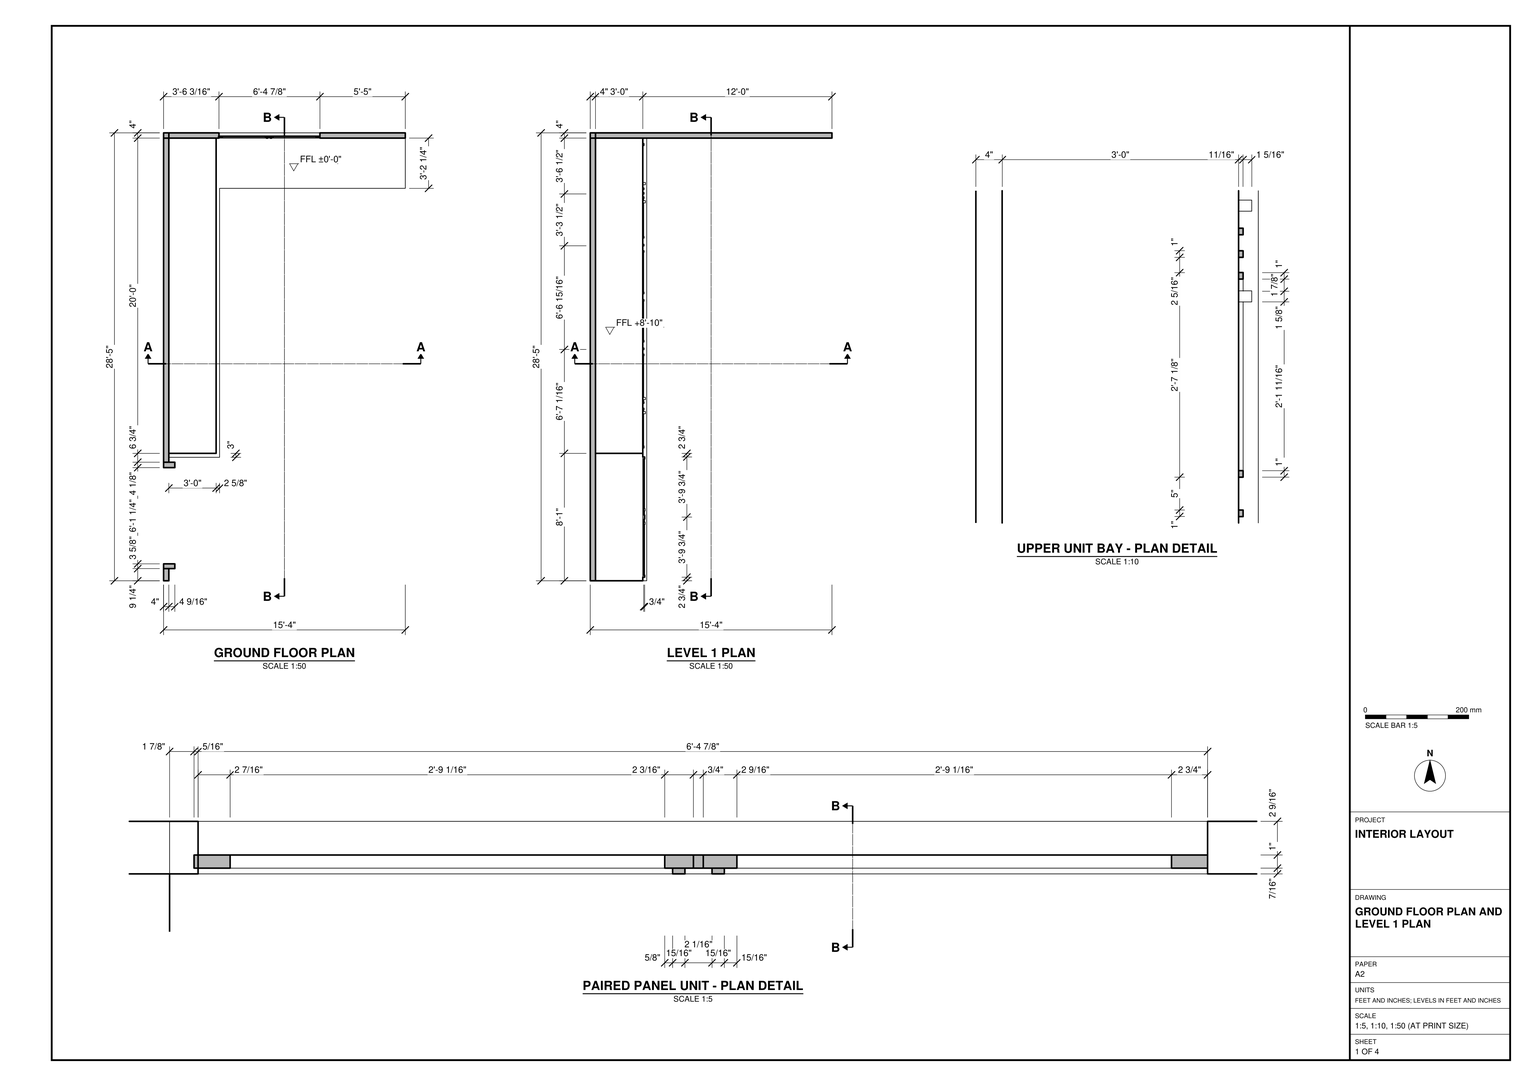
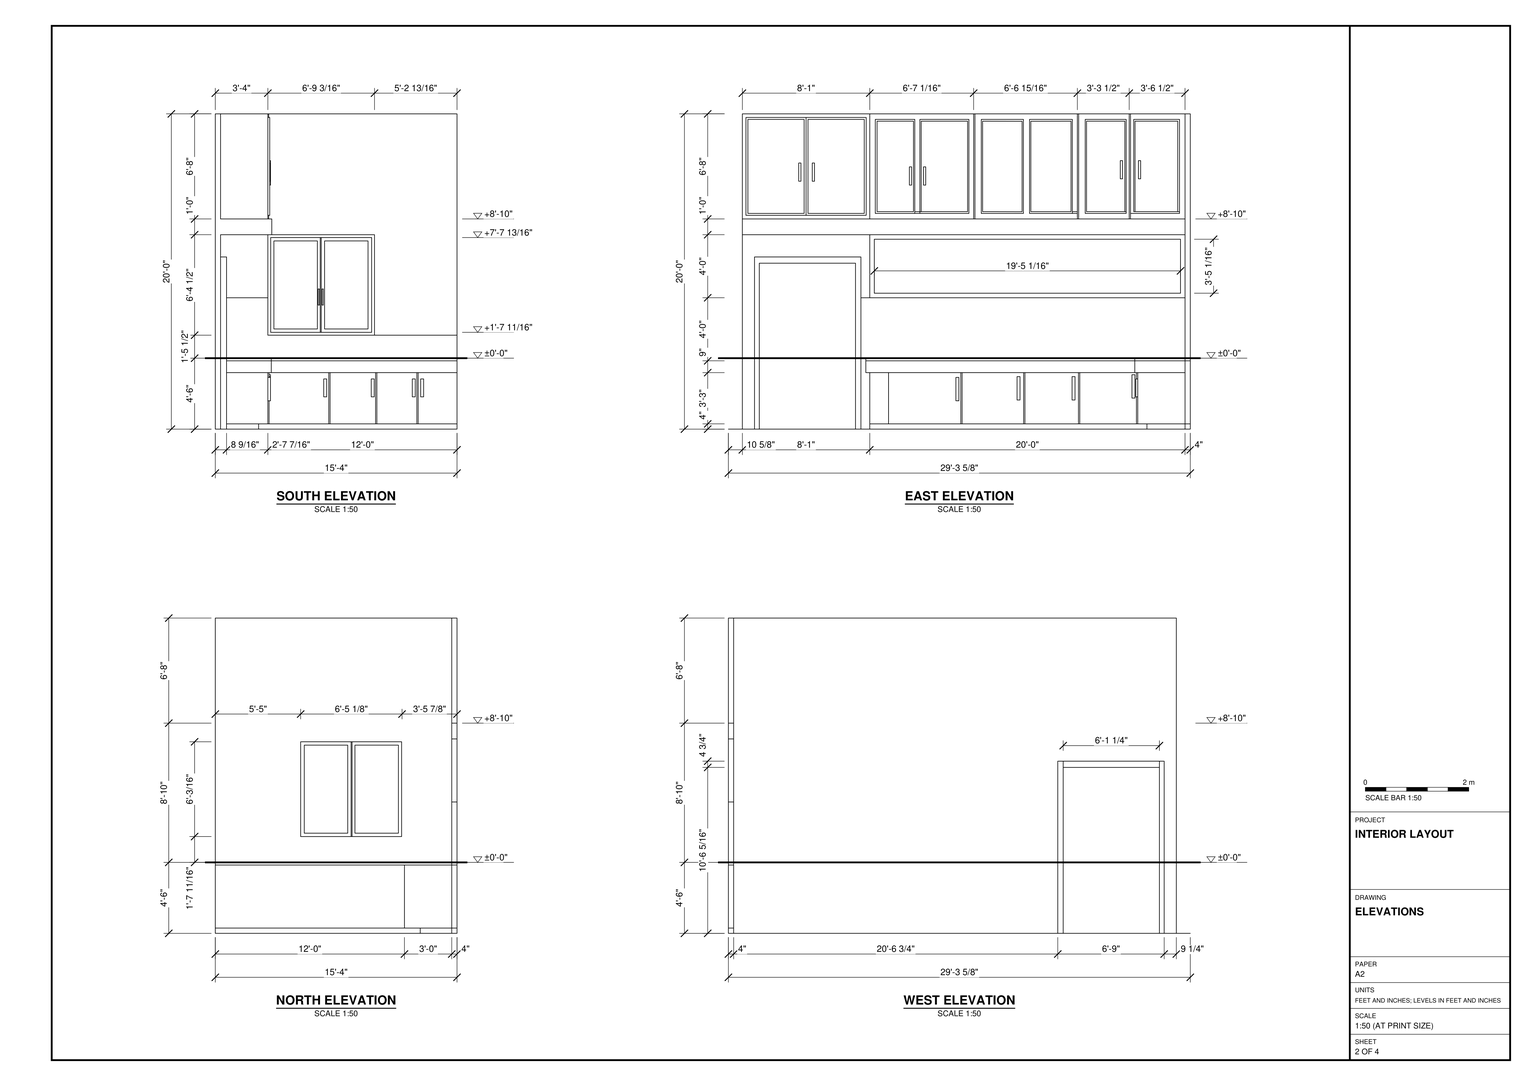
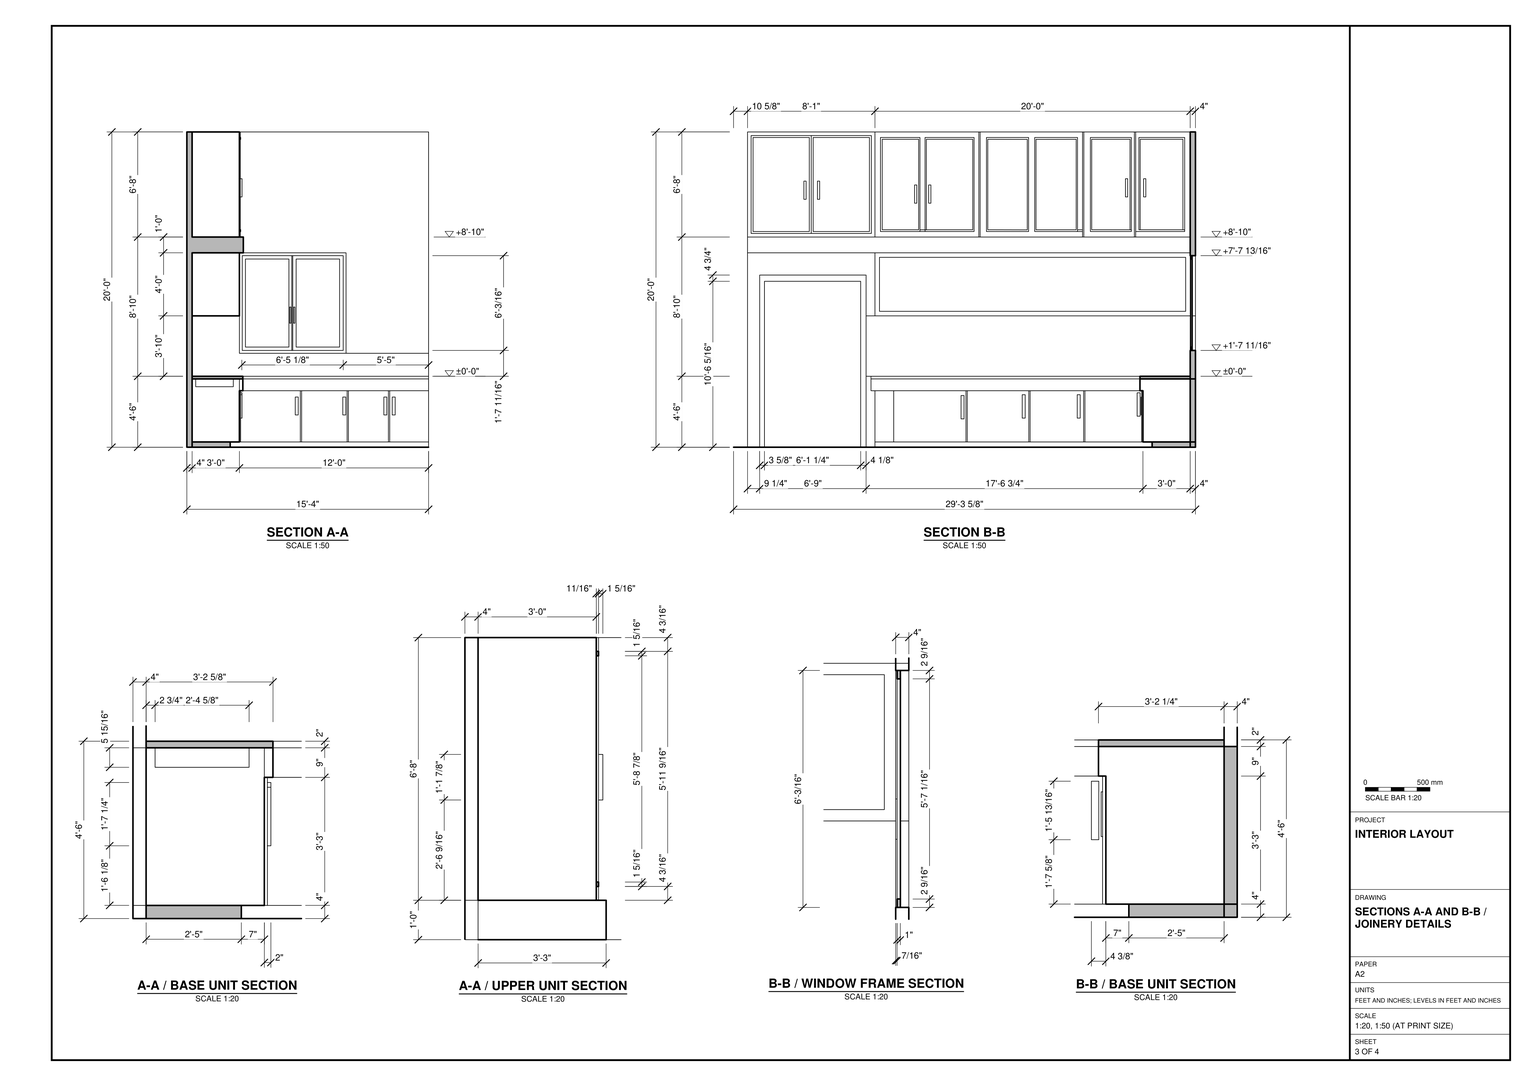
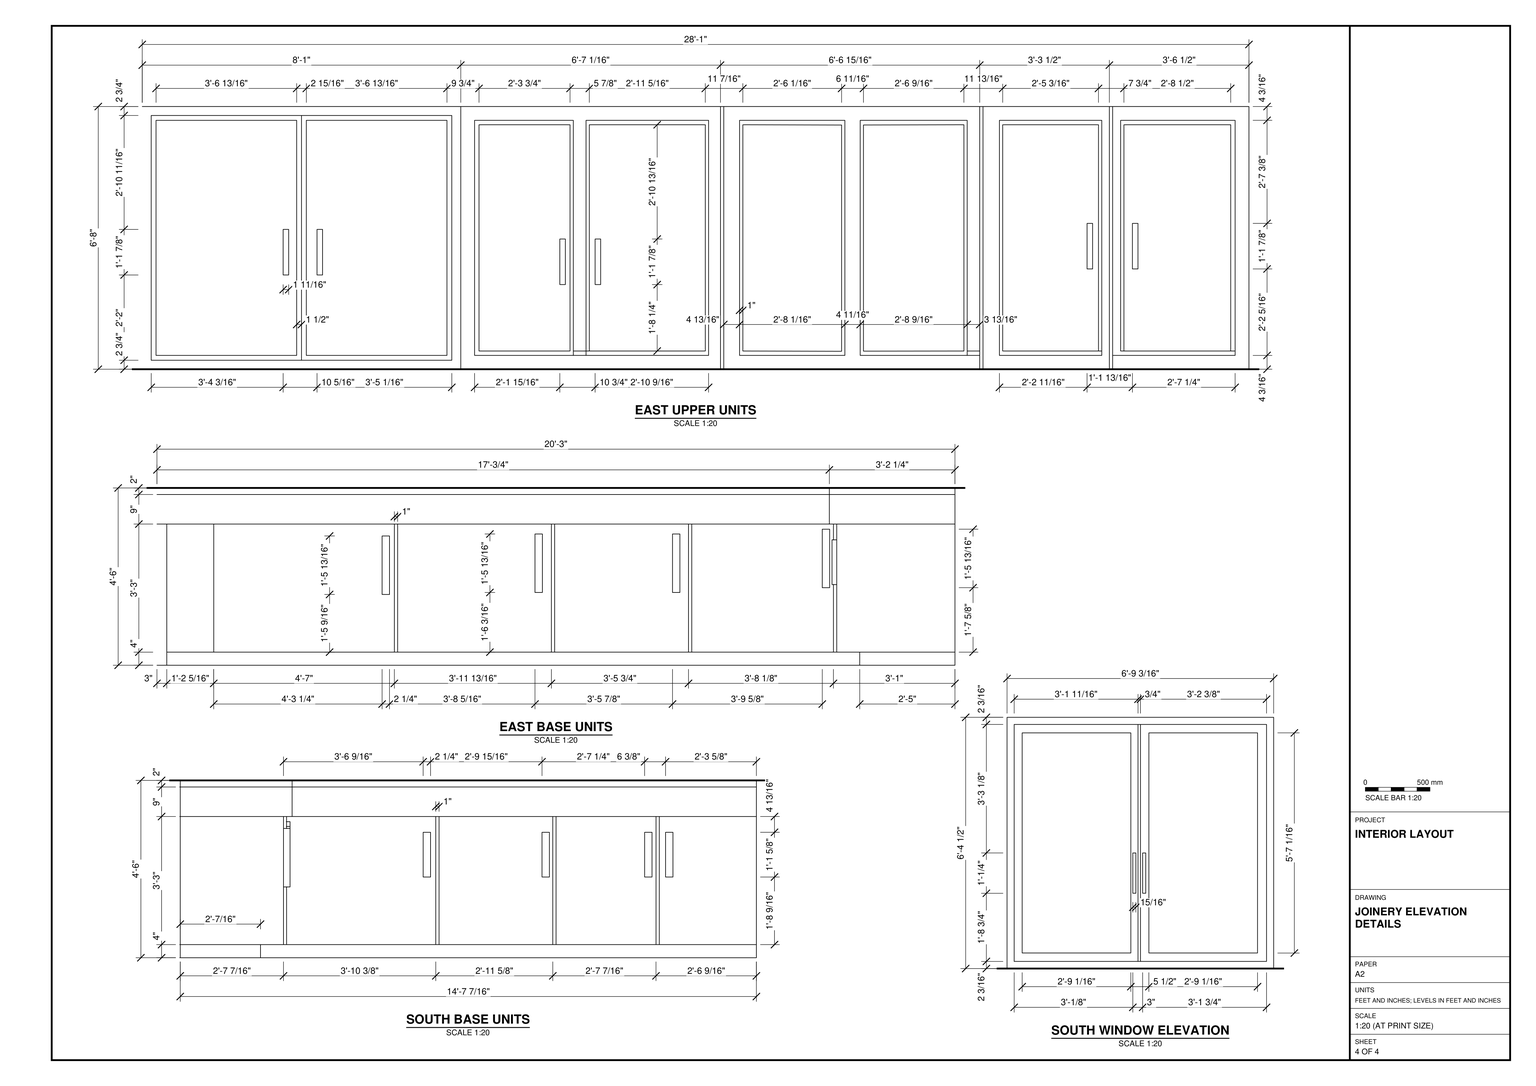
Build the interior fit-out in SketchUp from task_files/diagram_01.pdf. Work in feet and inches. Set the overall width to 15'-4", depth to 29'-3 5/8", and height to 20'-0". Use ±0'-0" as the ground-floor datum and +8'-10" as the Level 1 datum. The ground-floor datum aligns with the worktop, not the bottom of the model: the base units extend 4'-6" below it.

Form the corner with the two perpendicular 4" walls shown in plan. Fit the paired framed window in the short wall above the worktop. On the long wall, leave the tall framed opening near the free end and place the long horizontal framed panel above the base cabinets. Turn the worktop and base units around the inside corner, following the sections for the top overhangs and recessed plinths. Above the long wall run, model the projecting support slab and the upper cabinets. Use the east elevation to lay out the cabinet bays, framed fronts and pulls rather than dividing the run into equal bays.

Keep shell elements such as walls and slabs separate from one another, make each joinery or furniture piece a separate group or component, and use components for repeated parts. Any decor or loose items may be suitable library components. Save one SketchUp model as output_files/l_shaped_interior_fit_out_with_base_and_upper_cabinets.skp.

# SketchUp Ruby script. Lengths in inches.
U = 1.inch
M = Sketchup.active_model
def pt(a) = Geom::Point3d.new(a.map { |v| v * U })
def face(e, loops, mat)
  f = e.add_face(loops[0].map { |a| pt(a) })
  loops[1..].each { |l| e.add_face(l.map { |a| pt(a) }).erase! }
  f.material = f.back_material = mat if mat
  f
end
# faces: each face lists its corners as indices into pts; further lists are holes
def faces(e, pts, list, mat = nil) = list.each { |f| face(e, (f[0].is_a?(Array) ? f : [f]).map { |l| l.map { |i| pts[i] } }, mat) }
# xy, xz, yz: faces in a plane at the given z, y or x. An outline is a flat list of corners, or four numbers for a rectangle; further outlines are holes
def ring(l) = l.size == 4 ? [[l[0], l[1]], [l[2], l[1]], [l[2], l[3]], [l[0], l[3]]] : l.each_slice(2).to_a
def flat(e, list, mat, &to3) = list.each { |f| face(e, (f[0].is_a?(Array) ? f : [f]).map { |l| ring(l).map { |u, v| to3.(u, v) } }, mat) }
def xy(e, z, list, mat = nil) = flat(e, list, mat) { |x, y| [x, y, z] }
def xz(e, y, list, mat = nil) = flat(e, list, mat) { |x, z| [x, y, z] }
def yz(e, x, list, mat = nil) = flat(e, list, mat) { |y, z| [x, y, z] }
def lines(e, pts, list) = list.each { |a, b| e.add_line(pt(pts[a]), pt(pts[b])) }
# prism: a flat outline (further loops are holes) pulled along v
def prism(e, loops, v, mat = nil)
  f = face(e, loops, mat); d = Geom::Vector3d.new(v.map { |x| x * U })
  f.pushpull(f.normal.samedirection?(d) ? d.length : -d.length)
end
def box(e, o, s, mat = nil) = prism(e, [[o, [o[0] + s[0], o[1], o[2]], [o[0] + s[0], o[1] + s[1], o[2]], [o[0], o[1] + s[1], o[2]]]], [0, 0, s[2]], mat)
def at(x, y, z, deg = 0) = Geom::Transformation.translation(pt([x, y, z])) * Geom::Transformation.rotation(ORIGIN, Z_AXIS, deg.degrees)
def axes(o, x, y, z) = Geom::Transformation.new([*x, 0, *y, 0, *z, 0, *pt(o).to_a, 1])
def part(name) = M.definitions.add(name)
# library, detail: a bought-in or finely detailed component or shape, given as its bounding box
def library(name, o, s) = part(name).tap { |d| box(d.entities, o, s) }
def detail(e, o, s) = box(e.add_group.entities, o, s)
def put(e, d, t, mat = nil) = e.add_instance(d, t).tap { |i| i.material = mat if mat }
def group(e, t, mat = nil) = e.add_group.tap { |g| g.transformation = t; g.material = mat if mat }.entities
root = M.entities
M.materials.add("[0123_DarkMagenta]").color = [119, 35, 134]
M.materials.add("[Color C08]").color = [102, 51, 0]
M.materials.add("[Color K08]").color = [81, 11, 69]
M.materials.add("[Color M00]").color = [255, 255, 255]
M.materials.add("[Field Square Tile]").color = [217, 201, 169]
M.materials.add("[Granite Dark Gray]").color = [69, 68, 68]
M.materials.add("[Steel Brushed Stainless]").color = [183, 187, 190]
M.materials.add("[Stone Brushed Khaki]").color = [226, 197, 133]
M.materials.add("[Translucent Glass Gray]").color = [128, 128, 128]
M.materials["[Translucent Glass Gray]"].alpha = 0.5
xy(root,0,[[0,19.89,8.5625,23.52],[0,96.77,8.5625,100.89]])
xy(root,0,[[0,10.625,4,19.89],[0,100.89,4,347.625],[4,107.625,4,347.625,28,347.625,28,323.625,33,323.625,33,107.625],[33,318.625,33,323.625,28,323.625,28,347.625,184,347.625,184,318.625],[0,347.625,4,351.625],
  [4,347.625,28,351.625],[28,347.625,184,351.625]],"[Color M00]")
xy(root,0,[[4,0,4,19.89,8.5625,19.89,8.5625,23.52,0,23.52,0,96.77,8.5625,96.77,8.5625,100.89,4,100.89,4,107.625,33,107.625,33,318.625,184,318.625,184,0]],"[Stone Brushed Khaki]")
xy(root,4,[[33,107.625,40,318.625],[40,176.92,40.9375,177.92],[40,311.625,184,318.625]],"[Color K08]")
xy(root,4,[[4,107.625,4,347.625,28,347.625,28,323.625,33,323.625,33,107.625],[40,224.74,40.9375,225.74],[40,266.49,40.9375,267.49],[86.375,310.625,87.375,311.625],[122,310.625,123,311.625],
  [153.4375,310.625,154.4375,311.625],[33,318.625,33,323.625,28,323.625,28,347.625,40,347.625,40,318.625],[40,318.625,184,347.625],[0,347.625,4,351.625],[4,347.625,28,351.625],
  [28,347.625,40,351.625],[40,347.625,184,351.625]],"[Color M00]")
xy(root,21.56,[[40,173.19,42,175.44]],"[Steel Brushed Stainless]")
xy(root,22.17,[[40,219.74,42,221.99],[40,261.62,42,263.87]],"[Steel Brushed Stainless]")
xy(root,23.62,[[40,307.22,42,309.47]],"[Steel Brushed Stainless]")
xy(root,24.58,[[82.53,310.1875,84.78,311.625],[118.72,310.1875,120.97,311.625],[149.97,310.1875,152.22,311.625],[156.34,310.1875,158.59,311.625]],"[Steel Brushed Stainless]")
xy(root,38.2,[[82.53,310.1875,84.78,311.625],[118.72,310.1875,120.97,311.625],[149.97,310.1875,152.22,311.625],[156.34,310.1875,158.59,311.625]],"[Steel Brushed Stainless]")
xy(root,39.37,[[40,173.19,42,175.44]],"[Steel Brushed Stainless]")
xy(root,39.98,[[40,219.74,42,221.99],[40,261.62,42,263.87]],"[Steel Brushed Stainless]")
xy(root,41.43,[[40,307.22,42,309.47]],"[Steel Brushed Stainless]")
xy(root,43,[[40,176.92,40.9375,177.92]],"[Color K08]")
xy(root,43,[[4,104.625,42.625,107.625],[40,107.625,40,176.92,40.9375,176.92,40.9375,177.92,40,177.92,40,224.74,40.9375,224.74,40.9375,225.74,40,225.74,40,266.49,40.9375,266.49,40.9375,267.49,40,267.49,40,311.625,42.625,311.625,42.625,107.625],[40,224.74,40.9375,225.74],[40,266.49,40.9375,267.49],[42.625,309.375,42.625,311.625,86.375,311.625,86.375,310.625,87.375,310.625,87.375,311.625,122,311.625,122,310.625,123,310.625,123,311.625,153.4375,311.625,153.4375,310.625,154.4375,310.625,154.4375,311.625,184,311.625,184,309.375],
  [86.375,310.625,87.375,311.625],[122,310.625,123,311.625],[153.4375,310.625,154.4375,311.625]],"[Color M00]")
xy(root,46.0625,[[6.74,188.63,35.36,217.25]],"[Color M00]")
xy(root,52,[[4,104.625,4,347.625,184,347.625,184,309.375,42.625,309.375,42.625,104.625],[0,347.625,4,351.625],[4,347.625,40,351.625],[40,347.625,184,351.625]],"[Color M00]")
xy(root,54,[[[4,104.625,42.625,104.625,42.625,309.375,184,309.375,184,347.625,4,347.625],[6.74,188.63,35.36,217.25]]],"[Granite Dark Gray]")
xy(root,73.67,[[42.17,347.625,119.02,351.625]],"[Color M00]")
xy(root,100,[[4,107.625,40,347.625]],"[Color K08]")
xy(root,100,[[0,347.625,4,351.625]],"[Color M00]")
xy(root,126.3125,[[0,23.52,8.5625,96.77]],"[Color K08]")
xy(root,131.0625,[[0,19.89,4,23.52],[0,23.52,4,96.77],[0,96.77,4,100.89]])
xy(root,131.0625,[[4,19.89,8.5625,23.52],[4,23.52,8.5625,96.77],[4,96.77,8.5625,100.89]],"[Color K08]")
xy(root,145.83,[[42.17,347.625,119.02,351.625]],"[Color M00]")
xy(root,148,[[4,10.625,43,107.625],[4,107.625,40,347.625],[40,107.625,43,347.625],[0,347.625,4,351.625]],"[Color M00]")
xy(root,160,[[4,10.625,40,107.625],[40,10.625,43,10.625,43,347.625,40,347.625,40,306.12,40.6875,306.12,40.6875,305.12,40,305.12,40,266.64,40.6875,266.64,40.6875,265.64,40,265.64,40,187.71,40.6875,187.71,40.6875,186.71,40,186.71],[4,107.625,40,347.625],[40,186.71,40.6875,187.71],[40,186.71,40.6875,187.71],
  [40,265.64,40.6875,266.64],[40,265.64,40.6875,266.64],[40,305.12,40.6875,306.12],[40,305.12,40.6875,306.12],[0,347.625,4,351.625]],"[Color M00]")
xy(root,162.74,[[40,13.36,41.4375,59.125],[40,59.125,41.4375,104.89]],"[Color K08]")
xy(root,164.21,[[40.6875,14.83,41.4375,57.65],[40.6875,60.6,41.4375,103.42],[40,111.83,40.6875,141.89],[40,145.77,40.6875,183.08]],"[Color K08]")
xy(root,164.21,[[40,192.52,40.6875,224.58],[40,229.25,40.6875,261.83],[40,271.64,40.6875,302.81]],"[Color M00]")
xy(root,165.55,[[40,113.18,40.6875,140.89],[40,146.77,40.6875,182.08],[40,272.64,40.6875,301.81]],"[Color K08]")
xy(root,165.55,[[40,145.77,40.6875,146.77],[40,301.81,40.6875,302.81],[40,308.56,40.6875,309.56],[40,342.07,40.6875,343.42]],"[Color M00]")
xy(root,185.78,[[40,137.78,42,139.47],[40,148.53,42,150.22]],"[Steel Brushed Stainless]")
xy(root,188.71,[[40.6875,53.54,41.8125,55.22],[40.6875,63.85,41.8125,65.54]],"[Steel Brushed Stainless]")
xy(root,190.54,[[40,298.33,42,300.02],[40,312.14,42,313.83]],"[Steel Brushed Stainless]")
xy(root,199.65,[[40,137.78,42,139.47],[40,148.53,42,150.22]],"[Steel Brushed Stainless]")
xy(root,202.58,[[40.6875,53.54,41.8125,55.22],[40.6875,63.85,41.8125,65.54]],"[Steel Brushed Stainless]")
xy(root,204.41,[[40,298.33,42,300.02],[40,312.14,42,313.83]],"[Steel Brushed Stainless]")
xy(root,234.45,[[40,113.18,40.6875,140.89],[40,146.77,40.6875,182.08],[40,272.64,40.6875,301.81],[40,309.56,40.6875,342.07]],"[Color M00]")
xy(root,235.79,[[40.6875,14.83,41.4375,57.65],[40.6875,60.6,41.4375,103.42],[40,111.83,40.6875,141.89],[40,145.77,40.6875,183.08],[40,192.52,40.6875,224.58]],"[Color K08]")
xy(root,235.79,[[40,229.25,40.6875,261.83],[40,271.64,40.6875,302.81],[40,308.56,40.6875,343.42]],"[Color M00]")
xy(root,237.26,[[40,13.36,41.4375,59.125],[40,59.125,41.4375,104.89]],"[Color K08]")
xy(root,240,[[4,10.625,40,107.625],[4,107.625,40,347.625],[40,186.71,40.6875,187.71]],"[Color K08]")
xy(root,240,[[0,10.625,4,347.625],[40,265.64,40.6875,266.64],[40,305.12,40.6875,306.12],[0,347.625,4,351.625],[4,347.625,184,351.625]],"[Color M00]")
xz(root,10.625,[[0,0,4,0,4,148,43,148,43,160,4,160,4,240,0,240]])
xz(root,10.625,[[4,160,40,240]],"[Color K08]")
xz(root,13.36,[[40,162.74,41.4375,237.26]],"[Color K08]")
xz(root,14.83,[[40.6875,164.21,41.4375,235.79]],"[Color K08]")
xz(root,19.89,[[0,0,4,131.0625]])
xz(root,19.89,[[4,0,8.5625,131.0625]],"[Color K08]")
xz(root,23.52,[[0,0,8.5625,126.3125]],"[Color K08]")
xz(root,53.54,[[40.6875,188.71,41.8125,202.58]],"[Steel Brushed Stainless]")
xz(root,55.22,[[40.6875,188.71,41.8125,202.58]],"[Steel Brushed Stainless]")
xz(root,57.65,[[40.6875,164.21,41.4375,235.79]],"[Color K08]")
xz(root,60.6,[[40.6875,164.21,41.4375,235.79]],"[Color K08]")
xz(root,63.85,[[40.6875,188.71,41.8125,202.58]],"[Steel Brushed Stainless]")
xz(root,65.54,[[40.6875,188.71,41.8125,202.58]],"[Steel Brushed Stainless]")
xz(root,96.77,[[0,0,8.5625,126.3125]],"[Color K08]")
xz(root,100.89,[[0,0,4,131.0625]])
xz(root,100.89,[[4,0,8.5625,131.0625]],"[Color K08]")
xz(root,103.42,[[40.6875,164.21,41.4375,235.79]],"[Color K08]")
xz(root,104.625,[[4,43,42.625,52]],"[Color M00]")
xz(root,104.625,[[4,52,42.625,54]],"[Granite Dark Gray]")
xz(root,104.89,[[40,162.74,41.4375,237.26]],"[Color K08]")
xz(root,107.625,[[4,100,40,148],[4,160,40,240]],"[Color K08]")
xz(root,107.625,[[4,0,33,4],[4,4,40,43]],"[Color M00]")
xz(root,111.83,[[40,164.21,40.6875,235.79]],"[Color K08]")
xz(root,113.18,[[40,165.55,40.6875,234.45]],"[Color K08]")
xz(root,137.78,[[40,185.78,42,199.65]],"[Steel Brushed Stainless]")
xz(root,139.47,[[40,185.78,42,199.65]],"[Steel Brushed Stainless]")
xz(root,140.89,[[40,165.55,40.6875,234.45]],"[Color K08]")
xz(root,141.89,[[40,164.21,40.6875,165.55],[40,165.55,40.6875,235.79]],"[Color K08]")
xz(root,145.77,[[40,164.21,40.6875,165.55],[40,165.55,40.6875,235.79]],"[Color K08]")
xz(root,146.77,[[40,165.55,40.6875,234.45]],"[Color K08]")
xz(root,148.53,[[40,185.78,42,199.65]],"[Steel Brushed Stainless]")
xz(root,150.22,[[40,185.78,42,199.65]],"[Steel Brushed Stainless]")
xz(root,173.19,[[40,21.56,42,39.37]],"[Steel Brushed Stainless]")
xz(root,175.44,[[40,21.56,42,39.37]],"[Steel Brushed Stainless]")
xz(root,176.92,[[40,4,40.9375,43]],"[Color K08]")
xz(root,177.92,[[40,4,40.9375,43]],"[Color K08]")
xz(root,182.08,[[40,165.55,40.6875,234.45]],"[Color K08]")
xz(root,183.08,[[40,164.21,40.6875,235.79]],"[Color K08]")
xz(root,186.71,[[40,160,40.6875,240]],"[Color K08]")
xz(root,187.71,[[40,160,40.6875,240]],"[Color K08]")
xz(root,188.63,[[6.74,46.0625,35.36,54]],"[Color M00]")
xz(root,192.52,[[40,164.21,40.6875,235.79]],"[Color K08]")
xz(root,193.52,[[40,165.55,40.6875,234.45]],"[Color K08]")
xz(root,217.25,[[6.74,46.0625,35.36,54]],"[Color M00]")
xz(root,219.74,[[40,22.17,42,39.98]],"[Steel Brushed Stainless]")
xz(root,221.99,[[40,22.17,42,39.98]],"[Steel Brushed Stainless]")
xz(root,223.58,[[40,165.47,40.6875,234.37]],"[Color K08]")
xz(root,224.58,[[40,164.21,40.6875,235.79]],"[Color K08]")
xz(root,224.74,[[40,4,40.9375,43]],"[Color K08]")
xz(root,225.74,[[40,4,40.9375,43]],"[Color K08]")
xz(root,229.25,[[40,164.21,40.6875,235.79]],"[Color K08]")
xz(root,261.62,[[40,22.17,42,39.98]],"[Steel Brushed Stainless]")
xz(root,261.83,[[40,164.21,40.6875,165.55],[40,165.55,40.6875,235.79]],"[Color K08]")
xz(root,263.87,[[40,22.17,42,39.98]],"[Steel Brushed Stainless]")
xz(root,265.64,[[40,160,40.6875,164.21],[40,164.21,40.6875,165.55],[40,165.55,40.6875,240]],"[Color K08]")
xz(root,266.49,[[40,4,40.9375,43]],"[Color K08]")
xz(root,266.64,[[40,160,40.6875,240]],"[Color K08]")
xz(root,267.49,[[40,4,40.9375,43]],"[Color K08]")
xz(root,271.64,[[40,164.21,40.6875,235.79]],"[Color K08]")
xz(root,272.64,[[40,165.55,40.6875,234.45]],"[Color K08]")
xz(root,298.33,[[40,190.54,42,204.41]],"[Steel Brushed Stainless]")
xz(root,300.02,[[40,190.54,42,204.41]],"[Steel Brushed Stainless]")
xz(root,301.81,[[40,165.55,40.6875,234.45]],"[Color K08]")
xz(root,302.81,[[40,164.21,40.6875,165.55],[40,165.55,40.6875,235.79]],"[Color K08]")
xz(root,305.12,[[40,160,40.6875,240]],"[Color K08]")
xz(root,306.12,[[40,160,40.6875,164.21],[40,164.21,40.6875,240]],"[Color K08]")
xz(root,307.22,[[40,23.62,42,41.43]],"[Steel Brushed Stainless]")
xz(root,308.56,[[40,165.55,40.6875,235.79]],"[Color K08]")
xz(root,309.375,[[42.625,43,184,52]],"[Color M00]")
xz(root,309.375,[[42.625,52,184,54]],"[Granite Dark Gray]")
xz(root,309.47,[[40,23.62,42,41.43]],"[Steel Brushed Stainless]")
xz(root,309.56,[[40,165.55,40.6875,234.45]],"[Color K08]")
xz(root,310.1875,[[82.53,24.58,84.78,38.2],[118.72,24.58,120.97,38.2],[149.97,24.58,152.22,38.2],[156.34,24.58,158.59,38.2]],"[Steel Brushed Stainless]")
xz(root,310.625,[[86.375,4,87.375,43],[122,4,123,43],[153.4375,4,154.4375,43]],"[Color K08]")
xz(root,311.625,[[[40,4,86.375,43],[82.53,24.58,84.78,38.2]],[[87.375,4,122,43],[118.72,24.58,120.97,38.2]],[[123,4,153.4375,43],[149.97,24.58,152.22,38.2]],[[154.4375,4,184,43],[156.34,24.58,158.59,38.2]]],"[Color K08]")
xz(root,311.625,[[86.375,4,87.375,43],[122,4,123,43],[153.4375,4,154.4375,43]],"[Color M00]")
xz(root,311.625,[[82.53,24.58,84.78,38.2],[118.72,24.58,120.97,38.2],[149.97,24.58,152.22,38.2],[156.34,24.58,158.59,38.2]],"[Steel Brushed Stainless]")
xz(root,312.14,[[40,190.54,42,204.41]],"[Steel Brushed Stainless]")
xz(root,313.83,[[40,190.54,42,204.41]],"[Steel Brushed Stainless]")
xz(root,318.625,[[33,0,184,4]],"[Color M00]")
xz(root,323.625,[[28,0,33,4]],"[Color M00]")
xz(root,342.07,[[40,165.55,40.6875,234.45]],"[Color K08]")
xz(root,343.42,[[40,165.55,40.6875,235.79]],"[Color M00]")
xz(root,347.625,[[[40,71.5,121.1875,148],[42.17,73.67,119.02,145.83]]],"[0123_DarkMagenta]")
xz(root,347.625,[[0,0,4,4],[4,0,28,4],[28,0,184,4],[0,4,4,52],[4,4,40,52],
  [40,4,184,52],[0,52,4,100],[4,52,40,54],[40,52,184,54],[121.1875,71.5,184,71.5,184,240,40,240,40,160,43,160,43,148,121.1875,148],
  [0,100,4,148],[4,100,40,148],[0,148,4,160],[4,148,43,160],[0,160,4,240],
  [4,160,40,240]],"[Color M00]")
xz(root,347.625,[[4,54,184,54,184,71.5,40,71.5,40,100,4,100]],"[Field Square Tile]")
xz(root,351.625,[[0,0,4,4],[4,0,28,4],[28,0,184,4],[0,4,4,52],[4,4,40,52],
  [40,4,184,52],[0,52,4,100],[[4,52,184,240],[42.17,73.67,119.02,145.83]],[0,100,4,148],[0,148,4,160],
  [0,160,4,240]],"[Color M00]")
yz(root,0,[[10.625,0,10.625,240,347.625,240,347.625,0,100.89,0,100.89,131.0625,19.89,131.0625,19.89,0],[19.89,0,23.52,131.0625],[96.77,0,100.89,131.0625],[23.52,126.3125,96.77,131.0625]])
yz(root,0,[[347.625,0,351.625,4],[347.625,4,351.625,52],[347.625,52,351.625,100],[347.625,100,351.625,148],[347.625,148,351.625,160],
  [347.625,160,351.625,240]],"[Color M00]")
yz(root,4,[[10.625,0,19.89,0,19.89,131.0625,100.89,131.0625,100.89,100,107.625,100,107.625,148,10.625,148],[100.89,0,107.625,0,107.625,43,104.625,43,104.625,54,100.89,54]])
yz(root,4,[[107.625,0,347.625,4],[347.625,0,351.625,4],[107.625,4,347.625,4,347.625,52,104.625,52,104.625,43,107.625,43],[347.625,4,351.625,52],[104.625,52,347.625,54],
  [347.625,52,351.625,100],[107.625,100,347.625,148],[347.625,100,351.625,148],[347.625,148,351.625,160],[10.625,160,107.625,240],
  [107.625,160,347.625,240],[347.625,160,351.625,240]],"[Color M00]")
yz(root,4,[[100.89,54,347.625,100]],"[Field Square Tile]")
yz(root,6.74,[[188.63,46.0625,217.25,54]],"[Color M00]")
yz(root,8.5625,[[19.89,0,23.52,0,23.52,126.3125,96.77,126.3125,96.77,0,100.89,0,100.89,131.0625,19.89,131.0625]],"[Color K08]")
yz(root,28,[[323.625,0,347.625,4],[347.625,0,351.625,4]],"[Color M00]")
yz(root,33,[[107.625,0,318.625,4],[318.625,0,323.625,4]],"[Color M00]")
yz(root,35.36,[[188.63,46.0625,217.25,54]],"[Color M00]")
yz(root,40,[[141.89,164.21,145.77,165.55]])
yz(root,40,[[[121.92,4,176.92,43],[173.19,21.56,175.44,39.37]],[176.92,4,177.92,43],[[177.92,4,224.74,43],[219.74,22.17,221.99,39.98]],[[225.74,4,266.49,43],[261.62,22.17,263.87,39.98]],[[267.49,4,311.625,43],[307.22,23.62,309.47,41.43]],
  [[107.625,100,347.625,148],[111.08,103.46,344.17,144.54]],[[10.625,160,107.625,240],[13.36,162.74,104.89,237.26]],[[107.625,160,186.71,240],[111.83,164.21,111.83,235.79,141.89,235.79,141.89,165.55,145.77,165.55,145.77,235.79,183.08,235.79,183.08,164.21]],[[187.71,160,265.64,160,265.64,164.21,229.25,164.21,229.25,235.79,261.83,235.79,261.83,165.55,265.64,165.55,265.64,240,187.71,240],[192.52,164.21,224.58,235.79]],[[266.64,160,305.12,240],[271.64,164.21,302.81,235.79]],
  [306.12,160,347.625,160,347.625,240,306.12,240,306.12,164.21,343.42,164.21,343.42,165.55,308.56,165.55,308.56,235.79,343.42,235.79,343.42,164.21,306.12,164.21],[[141.89,164.21,141.89,165.55,140.89,165.55,140.89,234.45,113.18,234.45,113.18,165.55,145.77,165.55,145.77,164.21],[137.78,185.78,139.47,199.65]],[261.83,164.21,265.64,165.55],[223.58,165.47,223.58,234.37,193.52,234.45,193.52,165.55],[[146.77,165.55,182.08,234.45],[148.53,185.78,150.22,199.65]],
  [[272.64,165.55,301.81,234.45],[298.33,190.54,300.02,204.41]],[[309.56,165.55,342.07,234.45],[312.14,190.54,313.83,204.41]]],"[Color K08]")
yz(root,40,[[107.625,4,121.92,43],[224.74,4,225.74,43],[266.49,4,267.49,43],[347.625,4,351.625,52],[186.71,160,187.71,240],
  [265.64,160,266.64,240],[305.12,160,306.12,240],[[111.83,164.21,141.89,235.79],[113.18,165.55,140.89,234.45]],[145.77,164.21,145.77,165.55,182.08,165.55,182.08,234.45,146.77,234.45,146.77,165.55,145.77,165.55,145.77,235.79,183.08,235.79,183.08,164.21],[[192.52,164.21,224.58,235.79],[223.58,165.47,223.58,234.37,193.52,234.45,193.52,165.55]],
  [271.64,164.21,271.64,235.79,302.81,235.79,302.81,165.55,301.81,165.55,301.81,234.45,272.64,234.45,272.64,165.55,302.81,165.55,302.81,164.21],[308.56,165.55,308.56,235.79,343.42,235.79,343.42,165.55,342.07,165.55,342.07,234.45,309.56,234.45,309.56,165.55]],"[Color M00]")
yz(root,40,[[173.19,21.56,175.44,39.37],[219.74,22.17,221.99,39.98],[261.62,22.17,263.87,39.98],[307.22,23.62,309.47,41.43],[137.78,185.78,139.47,199.65],
  [148.53,185.78,150.22,199.65],[298.33,190.54,300.02,204.41],[312.14,190.54,313.83,204.41]],"[Steel Brushed Stainless]")
yz(root,40,[[111.08,103.46,344.17,144.54],[229.25,164.21,261.83,235.79]],"[Translucent Glass Gray]")
yz(root,40.6875,[[186.71,160,187.71,240],[265.64,160,266.64,240],[305.12,160,306.12,240],[[14.83,164.21,57.65,235.79],[53.54,188.71,55.22,202.58]],[[60.6,164.21,103.42,235.79],[63.85,188.71,65.54,202.58]],
  [[111.83,164.21,141.89,235.79],[113.18,165.55,140.89,234.45]],[145.77,164.21,183.08,164.21,183.08,235.79,145.77,235.79,145.77,165.55,146.77,165.55,146.77,234.45,182.08,234.45,182.08,165.55,145.77,165.55],[[192.52,164.21,224.58,235.79],[223.58,165.47,193.52,165.55,193.52,234.45,223.58,234.37]],[[229.25,164.21,261.83,235.79],[230.25,165.51,230.25,234.38,260.83,234.45,260.83,165.55]],[271.64,164.21,302.81,164.21,302.81,165.55,272.64,165.55,272.64,234.45,301.81,234.45,301.81,165.55,302.81,165.55,302.81,235.79,271.64,235.79],
  [308.56,165.55,309.56,165.55,309.56,234.45,342.07,234.45,342.07,165.55,343.42,165.55,343.42,235.79,308.56,235.79]],"[Color K08]")
yz(root,40.6875,[[63.85,188.71,65.54,202.58]],"[Steel Brushed Stainless]")
yz(root,40.9375,[[176.92,4,177.92,43],[224.74,4,225.74,43],[266.49,4,267.49,43]],"[Color K08]")
yz(root,41.4375,[[[13.36,162.74,59.125,237.26],[14.83,164.21,57.65,235.79]],[[59.125,162.74,104.89,237.26],[60.6,164.21,103.42,235.79]]],"[Color K08]")
yz(root,41.8125,[[53.54,188.71,55.22,202.58]],"[Color M00]")
yz(root,41.8125,[[63.85,188.71,65.54,202.58]],"[Steel Brushed Stainless]")
yz(root,42,[[173.19,21.56,175.44,39.37],[219.74,22.17,221.99,39.98],[261.62,22.17,263.87,39.98],[307.22,23.62,309.47,41.43],[137.78,185.78,139.47,199.65],
  [148.53,185.78,150.22,199.65],[298.33,190.54,300.02,204.41],[312.14,190.54,313.83,204.41]],"[Steel Brushed Stainless]")
yz(root,42.17,[[347.625,73.67,351.625,100],[347.625,100,351.625,145.83]],"[Color M00]")
yz(root,42.625,[[104.625,43,309.375,52]],"[Color M00]")
yz(root,42.625,[[104.625,52,309.375,54]],"[Granite Dark Gray]")
yz(root,43,[[10.625,148,347.625,160]],"[Color M00]")
yz(root,82.53,[[310.1875,24.58,311.625,38.2]],"[Steel Brushed Stainless]")
yz(root,84.78,[[310.1875,24.58,311.625,38.2]],"[Steel Brushed Stainless]")
yz(root,86.375,[[310.625,4,311.625,43]],"[Color K08]")
yz(root,87.375,[[310.625,4,311.625,43]],"[Color K08]")
yz(root,118.72,[[310.1875,24.58,311.625,38.2]],"[Steel Brushed Stainless]")
yz(root,119.02,[[347.625,73.67,351.625,145.83]],"[Color M00]")
yz(root,120.97,[[310.1875,24.58,311.625,38.2]],"[Steel Brushed Stainless]")
yz(root,122,[[310.625,4,311.625,43]],"[Color K08]")
yz(root,123,[[310.625,4,311.625,43]],"[Color K08]")
yz(root,149.97,[[310.1875,24.58,311.625,38.2]],"[Steel Brushed Stainless]")
yz(root,152.22,[[310.1875,24.58,311.625,38.2]],"[Steel Brushed Stainless]")
yz(root,153.4375,[[310.625,4,311.625,43]],"[Color K08]")
yz(root,154.4375,[[310.625,4,311.625,43]],"[Color K08]")
yz(root,156.34,[[310.1875,24.58,311.625,38.2]],"[Steel Brushed Stainless]")
yz(root,158.59,[[310.1875,24.58,311.625,38.2]],"[Steel Brushed Stainless]")
yz(root,184,[[311.625,4,347.625,43]],"[0123_DarkMagenta]")
yz(root,184,[[318.625,0,347.625,4],[347.625,0,351.625,4],[347.625,4,351.625,52],[309.375,43,347.625,52],[347.625,52,351.625,240]],"[Color M00]")
yz(root,184,[[309.375,52,347.625,54]],"[Granite Dark Gray]")
p = [[40,223.58,165.47],[40,193.52,165.55],[40.6875,193.52,165.55],[40.6875,223.58,165.47],[40,193.52,234.45],[40,223.58,234.37],
  [40.6875,223.58,234.37],[40.6875,193.52,234.45],[40,347.625,100],[40,351.625,100],[40,347.625,148],[40,351.625,148],
  [40,260.83,234.45],[40.6875,260.83,234.45],[40,230.25,234.38],[40.6875,230.25,234.38],[40,260.83,165.55],[40.6875,260.83,165.55],
  [40,230.25,165.51],[40.6875,230.25,165.51],[40,230.25,234.36],[40.6875,230.25,234.36]]
faces(root,p,[[0,1,2,3]],"[Color K08]")
faces(root,p,[[4,5,6,7]],"[Color M00]")
lines(root,p,[[8,9],[10,11],[12,13],[14,15],[16,17],[18,19],[20,21]])
g1 = group(root,at(41.86,347.625,73.67))
xy(g1,0,[[0,0.4375,38.02,1.4375],[38.02,0.4375,38.77,1.4375],[38.77,0.4375,77.16,1.4375]],"[Color K08]")
xy(g1,2.57,[[2.75,0.4375,35.83,1.4375],[41.32,0.4375,74.41,1.4375]],"[Color K08]")
xy(g1,20.75,[[36.43,0,37.37,0.4375],[39.43,0,40.37,0.4375]],"[Steel Brushed Stainless]")
xy(g1,33.03,[[36.43,0,37.37,0.4375],[39.43,0,40.37,0.4375]],"[Steel Brushed Stainless]")
xy(g1,69.59,[[2.75,0.4375,35.83,1.4375],[41.32,0.4375,74.41,1.4375]],"[Color K08]")
xy(g1,72.16,[[0,0.4375,38.02,1.4375],[38.02,0.4375,38.77,1.4375],[38.77,0.4375,77.16,1.4375]],"[Color K08]")
xz(g1,0,[[36.43,20.75,37.37,33.03],[39.43,20.75,40.37,33.03]],"[Steel Brushed Stainless]")
xz(g1,0.4375,[[[0,0,38.02,72.16],[2.75,2.57,35.83,69.59],[36.43,20.75,37.37,33.03]],[38.02,0,38.77,72.16],[[38.77,0,77.16,72.16],[41.32,2.57,74.41,69.59],[39.43,20.75,40.37,33.03]]],"[Color K08]")
xz(g1,0.4375,[[36.43,20.75,37.37,33.03],[39.43,20.75,40.37,33.03]],"[Steel Brushed Stainless]")
xz(g1,1.4375,[[[0,0,38.02,72.16],[2.75,2.57,35.83,69.59]],[38.02,0,38.77,72.16],[[38.77,0,77.16,72.16],[41.32,2.57,74.41,69.59]]],"[Color K08]")
xz(g1,1.4375,[[2.75,2.57,35.83,69.59],[41.32,2.57,74.41,69.59]],"[Translucent Glass Gray]")
yz(g1,0,[[0.4375,0,1.4375,72.16]],"[Color K08]")
yz(g1,2.75,[[0.4375,2.57,1.4375,69.59]],"[Color K08]")
yz(g1,35.83,[[0.4375,2.57,1.4375,69.59]],"[Color K08]")
yz(g1,36.43,[[0,20.75,0.4375,33.03]],"[Steel Brushed Stainless]")
yz(g1,37.37,[[0,20.75,0.4375,33.03]],"[Steel Brushed Stainless]")
yz(g1,38.02,[[0.4375,0,1.4375,72.16]],"[Color C08]")
yz(g1,38.77,[[0.4375,0,1.4375,72.16]],"[Color C08]")
yz(g1,39.43,[[0,20.75,0.4375,33.03]],"[Steel Brushed Stainless]")
yz(g1,40.37,[[0,20.75,0.4375,33.03]],"[Steel Brushed Stainless]")
yz(g1,41.32,[[0.4375,2.57,1.4375,69.59]],"[Color K08]")
yz(g1,74.41,[[0.4375,2.57,1.4375,69.59]],"[Color K08]")
yz(g1,77.16,[[0.4375,0,1.4375,72.16]],"[Color K08]")
